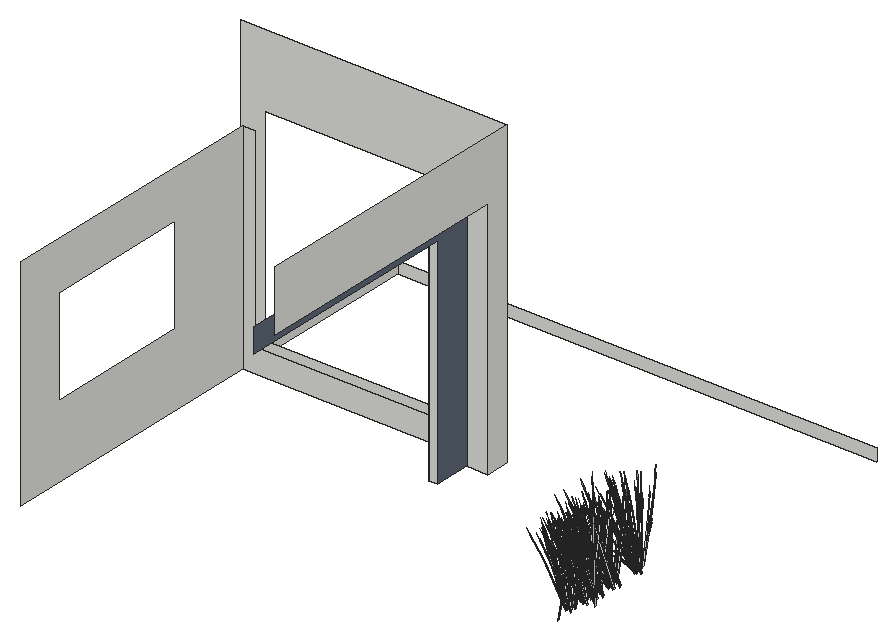
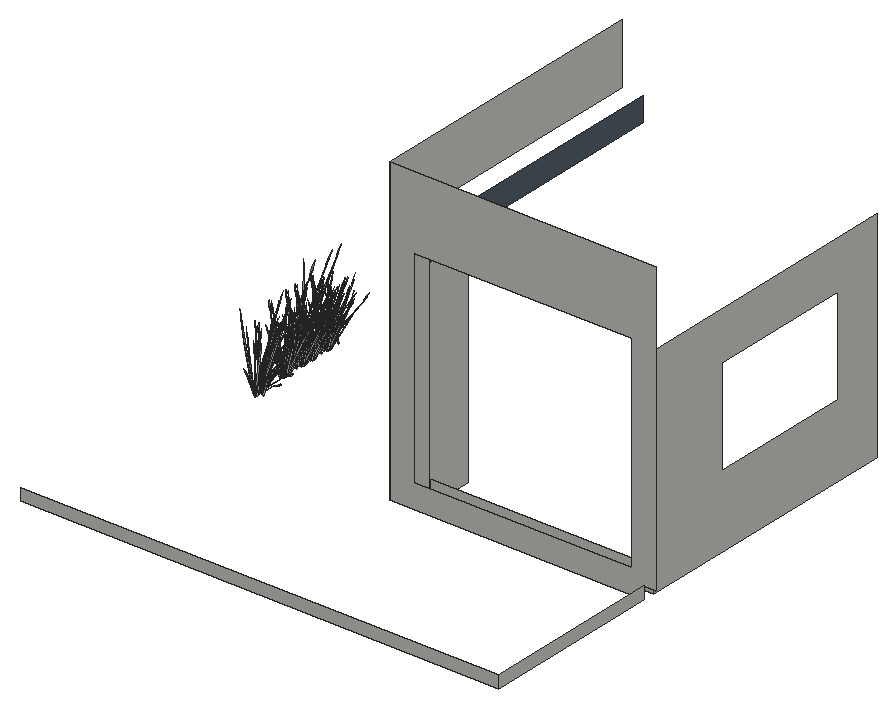
# SketchUp Ruby script. Lengths in inches.
U = 1.inch
M = Sketchup.active_model
def pt(a) = Geom::Point3d.new(a.map { |v| v * U })
def face(e, loops, mat)
  f = e.add_face(loops[0].map { |a| pt(a) })
  loops[1..].each { |l| e.add_face(l.map { |a| pt(a) }).erase! }
  f.material = f.back_material = mat if mat
  f
end
# faces: each face lists its corners as indices into pts; further lists are holes
def faces(e, pts, list, mat = nil) = list.each { |f| face(e, (f[0].is_a?(Array) ? f : [f]).map { |l| l.map { |i| pts[i] } }, mat) }
# xy, xz, yz: faces in a plane at the given z, y or x. An outline is a flat list of corners, or four numbers for a rectangle; further outlines are holes
def ring(l) = l.size == 4 ? [[l[0], l[1]], [l[2], l[1]], [l[2], l[3]], [l[0], l[3]]] : l.each_slice(2).to_a
def flat(e, list, mat, &to3) = list.each { |f| face(e, (f[0].is_a?(Array) ? f : [f]).map { |l| ring(l).map { |u, v| to3.(u, v) } }, mat) }
def xy(e, z, list, mat = nil) = flat(e, list, mat) { |x, y| [x, y, z] }
def xz(e, y, list, mat = nil) = flat(e, list, mat) { |x, z| [x, y, z] }
def yz(e, x, list, mat = nil) = flat(e, list, mat) { |y, z| [x, y, z] }
def lines(e, pts, list) = list.each { |a, b| e.add_line(pt(pts[a]), pt(pts[b])) }
# prism: a flat outline (further loops are holes) pulled along v
def prism(e, loops, v, mat = nil)
  f = face(e, loops, mat); d = Geom::Vector3d.new(v.map { |x| x * U })
  f.pushpull(f.normal.samedirection?(d) ? d.length : -d.length)
end
def box(e, o, s, mat = nil) = prism(e, [[o, [o[0] + s[0], o[1], o[2]], [o[0] + s[0], o[1] + s[1], o[2]], [o[0], o[1] + s[1], o[2]]]], [0, 0, s[2]], mat)
def at(x, y, z, deg = 0) = Geom::Transformation.translation(pt([x, y, z])) * Geom::Transformation.rotation(ORIGIN, Z_AXIS, deg.degrees)
def axes(o, x, y, z) = Geom::Transformation.new([*x, 0, *y, 0, *z, 0, *pt(o).to_a, 1])
def part(name) = M.definitions.add(name)
# library, detail: a bought-in or finely detailed component or shape, given as its bounding box
def library(name, o, s) = part(name).tap { |d| box(d.entities, o, s) }
def detail(e, o, s) = box(e.add_group.entities, o, s)
def put(e, d, t, mat = nil) = e.add_instance(d, t).tap { |i| i.material = mat if mat }
def group(e, t, mat = nil) = e.add_group.tap { |g| g.transformation = t; g.material = mat if mat }.entities
root = M.entities
M.materials.add("Denim_03_1K").color = [93, 106, 119]
M.materials.add("LightPink_Translucent").color = [144, 107, 117]
M.materials["LightPink_Translucent"].alpha = 0.75
c1 = part("blade")
p = [[2.15,0.21,22],[0,0.17,0],[0.09,0.45,0],[2.18,0.31,22],[2.29,0.31,22],[0.38,0.45,0],
  [2.48,0.24,33],[2.49,0.24,33],[2.48,0.22,33]]
faces(c1.entities,p,[[0,1,2,3],[4,5,2,3],[6,3,4,7],[8,0,3,6]])
c2 = part("seeds")
p = [[0.3,-0.1,1.38],[-0.01,-0.03,1.59],[-0.01,-0.03,0.03],[0.14,-0.07,-0.07],[0.29,-0.03,3],[0.15,0.01,3.11]]
faces(c2.entities,p,[[0,1,2,3],[1,0,4,5]],"LightPink_Translucent")
c3 = part("blade with seeds")
put(c3.entities,c1,at(0,0,0))
put(c3.entities,c2,axes([2.4,0.25,30.99],[1.5799,-0.05474,1.17369],[-0.12525,1.92788,0.29478],[-0.07173,-0.02425,1.56792]))
xz(root,405,[[162,126,166.5,234]])
xz(root,423,[[166.5,126,177,246]])
xz(root,429,[[51,126,162,126,162,138,57,138,57,234,51,234]])
xz(root,435,[[[51,126,51,132,45,132,45,276,177,276,177,126],[57,138,165,240]]])
xz(root,525,[[51,126,288,132]])
yz(root,51,[[[291,126,429,234],[315,162,387,210]],[435,126,525,132]])
yz(root,162,[[405,126,429,234]])
yz(root,166.5,[[405,126,423,126,423,246,291,246,291,234,405,234]],"Denim_03_1K")
yz(root,177,[[423,126,435,126,435,276,291,276,291,246,423,246]])
put(root,c3,axes([268.35,357.15,126.52],[0.37107,-0.01478,1.71376],[-0.24616,0.64047,0.13857],[-0.5288,-0.03961,0.73262]))
put(root,c3,axes([268.35,366.98,126.55],[0.37107,-0.01478,1.71376],[-0.24616,0.64047,0.13857],[-0.5288,-0.03961,0.73262]))
put(root,c3,axes([268.35,372.59,126.42],[0.37107,-0.01478,1.71376],[-0.24616,0.64047,0.13857],[-0.5288,-0.03961,0.73262]))
put(root,c3,axes([268.35,382.95,126.46],[0.37107,-0.01478,1.71376],[-0.24616,0.64047,0.13857],[-0.5288,-0.03961,0.73262]))
put(root,c3,axes([268.35,400.0625,125.79],[0.37107,-0.01478,1.71376],[-0.24616,0.64047,0.13857],[-0.5288,-0.03961,0.73262]))
put(root,c3,axes([268.51,358.28,126.52],[0.31041,-0.13801,1.71376],[0.26133,0.63772,0.13857],[-0.48731,0.14413,0.73262]))
put(root,c3,axes([268.51,368.1,126.55],[0.31041,-0.13801,1.71376],[0.26133,0.63772,0.13857],[-0.48731,0.14413,0.73262]))
put(root,c3,axes([268.51,373.72,126.42],[0.31041,-0.13801,1.71376],[0.26133,0.63772,0.13857],[-0.48731,0.14413,0.73262]))
put(root,c3,axes([268.51,384.08,126.46],[0.31041,-0.13801,1.71376],[0.26133,0.63772,0.13857],[-0.48731,0.14413,0.73262]))
put(root,c3,axes([268.51,401.19,125.79],[0.31041,-0.13801,1.71376],[0.26133,0.63772,0.13857],[-0.48731,0.14413,0.73262]))
put(root,c3,axes([270.29,357.62,125.99],[0.25429,-0.09438,1.77064],[0.08769,0.65901,0.13857],[-0.5508,0.08745,0.63284]))
put(root,c3,axes([270.29,367.4375,126.02],[0.25429,-0.09438,1.77064],[0.08769,0.65901,0.13857],[-0.5508,0.08745,0.63284]))
put(root,c3,axes([270.29,373.05,125.89],[0.25429,-0.09438,1.77064],[0.08769,0.65901,0.13857],[-0.5508,0.08745,0.63284]))
put(root,c3,axes([270.29,383.41,125.92],[0.25429,-0.09438,1.77064],[0.08769,0.65901,0.13857],[-0.5508,0.08745,0.63284]))
put(root,c3,axes([267.56,400.97,126.63],[-0.14609,0.08471,1.74944],[0.01243,0.61893,-0.27667],[-0.33486,0.08049,0.14031]))
put(root,c3,axes([269.46,366.38,127.66],[-0.89428,-0.01571,-0.71045],[0.06006,-0.66153,0.08574],[-0.37886,-0.06981,1.00501]))
put(root,c3,axes([269.46,382.36,127.5625],[-0.89428,-0.01571,-0.71045],[0.06006,-0.66153,0.08574],[-0.37886,-0.06981,1.00501]))
put(root,c3,axes([268.03,357.7,127.17],[-0.74348,-0.18202,-0.35414],[0.21685,-0.53102,0.4572],[-0.29933,0.04869,0.87481]))
put(root,c3,axes([268.03,367.53,127.2],[-0.74348,-0.18202,-0.35414],[0.21685,-0.53102,0.4572],[-0.29933,0.04869,0.87481]))
put(root,c3,axes([268.03,373.14,127.07],[-0.74348,-0.18202,-0.35414],[0.21685,-0.53102,0.4572],[-0.29933,0.04869,0.87481]))
put(root,c3,axes([268.03,383.5,127.11],[-0.74348,-0.18202,-0.35414],[0.21685,-0.53102,0.4572],[-0.29933,0.04869,0.87481]))
put(root,c3,axes([269.05,365.95,126.55],[0.3323,0.11241,1.71376],[-0.68769,0.4716,0.13857],[-0.42861,-0.21275,0.73262]))
put(root,c3,axes([269.05,371.5625,126.42],[0.3323,0.11241,1.71376],[-0.68769,0.4716,0.13857],[-0.42861,-0.21275,0.73262]))
put(root,c3,axes([269.05,381.92,126.46],[0.3323,0.11241,1.71376],[-0.68769,0.4716,0.13857],[-0.42861,-0.21275,0.73262]))
put(root,c3,axes([269.05,399.04,125.79],[0.3323,0.11241,1.71376],[-0.68769,0.4716,0.13857],[-0.42861,-0.21275,0.73262]))
put(root,c3,axes([265.93,401.59,126.625],[0.11417,0.0175,1.77383],[0.35319,0.57649,-0.16761],[-0.23371,0.15131,0.31391]))
put(root,c3,axes([268.54,357.97,127.33],[-0.24236,0.59349,-0.51099],[-0.83094,-0.20343,-0.3958],[-0.33455,0.05442,0.97773]))
put(root,c3,axes([268.54,367.8,127.36],[-0.24236,0.59349,-0.51099],[-0.83094,-0.20343,-0.3958],[-0.33455,0.05442,0.97773]))
put(root,c3,axes([268.54,373.41,127.23],[-0.24236,0.59349,-0.51099],[-0.83094,-0.20343,-0.3958],[-0.33455,0.05442,0.97773]))
put(root,c3,axes([268.54,383.77,127.26],[-0.24236,0.59349,-0.51099],[-0.83094,-0.20343,-0.3958],[-0.33455,0.05442,0.97773]))
put(root,c3,axes([269.17,366.51,127.36],[-0.6496,0.4322,-0.51099],[-0.5689,-0.45657,-0.3958],[-0.33005,-0.06576,0.97773]))
put(root,c3,axes([269.17,372.13,127.23],[-0.6496,0.4322,-0.51099],[-0.5689,-0.45657,-0.3958],[-0.33005,-0.06576,0.97773]))
put(root,c3,axes([269.17,382.49,127.26],[-0.6496,0.4322,-0.51099],[-0.5689,-0.45657,-0.3958],[-0.33005,-0.06576,0.97773]))
put(root,c3,axes([268.25,398.39,126.625],[0.06632,0.06511,1.77383],[-0.31973,0.58531,-0.16761],[-0.32381,0.00424,0.31391]))
put(root,c3,axes([268.99,398,126.63],[-0.19249,-0.00461,1.74944],[-0.61281,0.46055,-0.27667],[-0.32697,-0.0941,0.14031]))
put(root,c3,axes([268.2,400.55,126.65],[0.25275,-0.59491,0.48003],[0.83094,0.20343,0.3958],[-0.32677,0.03575,0.9933]))
put(root,c3,axes([268.5,357.47,127.68],[0.45012,0.59081,-0.1216],[-0.79888,0.29033,-0.67495],[-0.33665,0.07795,1.02557]))
put(root,c3,axes([268.5,372.9,127.58],[0.45012,0.59081,-0.1216],[-0.79888,0.29033,-0.67495],[-0.33665,0.07795,1.02557]))
put(root,c3,axes([268.5,383.26,127.61],[0.45012,0.59081,-0.1216],[-0.79888,0.29033,-0.67495],[-0.33665,0.07795,1.02557]))
put(root,c3,axes([268.5,400.375,126.95],[0.45012,0.59081,-0.1216],[-0.79888,0.29033,-0.67495],[-0.33665,0.07795,1.02557]))
put(root,c3,axes([269.51,356.24,127.68],[-0.0479,0.66354,-0.1216],[-0.90696,-0.01814,-0.67495],[-0.3493,-0.04609,1.02557]))
put(root,c3,axes([269.51,371.68,127.58],[-0.0479,0.66354,-0.1216],[-0.90696,-0.01814,-0.67495],[-0.3493,-0.04609,1.02557]))
put(root,c3,axes([269.51,382.04,127.61],[-0.0479,0.66354,-0.1216],[-0.90696,-0.01814,-0.67495],[-0.3493,-0.04609,1.02557]))
put(root,c3,axes([269.51,399.15,126.95],[-0.0479,0.66354,-0.1216],[-0.90696,-0.01814,-0.67495],[-0.3493,-0.04609,1.02557]))
put(root,c3,axes([268.92,366.11,127.2],[-0.50902,-0.40851,-0.35414],[0.58122,-0.38671,0.4572],[-0.29531,-0.05884,0.87481]))
put(root,c3,axes([268.92,371.72,127.07],[-0.50902,-0.40851,-0.35414],[0.58122,-0.38671,0.4572],[-0.29531,-0.05884,0.87481]))
put(root,c3,axes([268.92,382.08,127.11],[-0.50902,-0.40851,-0.35414],[0.58122,-0.38671,0.4572],[-0.29531,-0.05884,0.87481]))
put(root,c3,axes([268.14,400.39,126.64],[-0.32857,-0.44488,0.0643],[0.59916,-0.21775,0.50621],[-0.26412,0.04296,0.77189]))
put(root,c3,axes([269.64,358.71,126.52],[0.22344,-0.20048,1.71376],[0.56419,0.54113,0.13857],[-0.38697,0.24643,0.73262]))
put(root,c3,axes([269.64,368.53,126.55],[0.22344,-0.20048,1.71376],[0.56419,0.54113,0.13857],[-0.38697,0.24643,0.73262]))
put(root,c3,axes([269.64,374.15,126.42],[0.22344,-0.20048,1.71376],[0.56419,0.54113,0.13857],[-0.38697,0.24643,0.73262]))
put(root,c3,axes([269.64,384.51,126.46],[0.22344,-0.20048,1.71376],[0.56419,0.54113,0.13857],[-0.38697,0.24643,0.73262]))
put(root,c3,axes([269.64,401.62,125.79],[0.22344,-0.20048,1.71376],[0.56419,0.54113,0.13857],[-0.38697,0.24643,0.73262]))
put(root,c3,axes([268.3,359.24,127.17],[-0.77872,0.09325,-0.35414],[-0.20563,-0.53305,0.4572],[-0.22316,0.14318,0.87481]))
put(root,c3,axes([268.3,369.06,127.2],[-0.77872,0.09325,-0.35414],[-0.20563,-0.53305,0.4572],[-0.22316,0.14318,0.87481]))
put(root,c3,axes([268.3,374.67,127.07],[-0.77872,0.09325,-0.35414],[-0.20563,-0.53305,0.4572],[-0.22316,0.14318,0.87481]))
put(root,c3,axes([268.3,385.03,127.11],[-0.77872,0.09325,-0.35414],[-0.20563,-0.53305,0.4572],[-0.22316,0.14318,0.87481]))
put(root,c3,axes([268.4,402.03,126.65],[-0.22187,-0.60049,0.48003],[0.87033,-0.10422,0.3958],[-0.25651,0.14123,0.9933]))
put(root,c3,axes([268.85,399.04,127.01],[0.7388,-0.48151,0.53763],[0.63717,0.51135,0.4433],[-0.34662,-0.08882,1.11249]))
put(root,c3,axes([268.23,401.91,126.64],[-0.61415,-0.2744,0.0643],[0.35756,-0.39076,0.50621],[-0.1969,0.12633,0.77189]))
put(root,c3,axes([269.48,359.2,126.52],[0.16657,-0.22426,1.71376],[0.69879,0.4641,0.13857],[-0.31524,0.28926,0.73262]))
put(root,c3,axes([269.48,369.03,126.55],[0.16657,-0.22426,1.71376],[0.69879,0.4641,0.13857],[-0.31524,0.28926,0.73262]))
put(root,c3,axes([269.48,374.64,126.42],[0.16657,-0.22426,1.71376],[0.69879,0.4641,0.13857],[-0.31524,0.28926,0.73262]))
put(root,c3,axes([269.48,385,126.46],[0.16657,-0.22426,1.71376],[0.69879,0.4641,0.13857],[-0.31524,0.28926,0.73262]))
put(root,c3,axes([269.48,402.11,125.79],[0.16657,-0.22426,1.71376],[0.69879,0.4641,0.13857],[-0.31524,0.28926,0.73262]))
put(root,c3,axes([268.81,400.56,126.97],[0.74348,0.18202,0.35414],[-0.21685,0.53102,-0.4572],[-0.29933,0.04869,0.87481]))
put(root,c3,axes([268.94,359.3,127.33],[0.22982,0.59576,-0.51099],[-0.87033,0.10422,-0.3958],[-0.24941,0.16002,0.97773]))
put(root,c3,axes([268.94,369.12,127.36],[0.22982,0.59576,-0.51099],[-0.87033,0.10422,-0.3958],[-0.24941,0.16002,0.97773]))
put(root,c3,axes([268.94,374.73,127.23],[0.22982,0.59576,-0.51099],[-0.87033,0.10422,-0.3958],[-0.24941,0.16002,0.97773]))
put(root,c3,axes([268.94,385.1,127.26],[0.22982,0.59576,-0.51099],[-0.87033,0.10422,-0.3958],[-0.24941,0.16002,0.97773]))
put(root,c3,axes([269.19,399.04,126.64],[0.04505,-0.49615,0.0643],[0.68022,0.0136,0.50621],[-0.26056,-0.05192,0.77189]))
put(root,c3,axes([267.58,403.28,126.63],[-0.02224,0.12912,1.74944],[0.63107,0.44917,-0.27667],[-0.16521,0.21241,0.14031]))
put(root,c3,axes([271.28,398.18,127.34],[-0.59706,0.6255,-0.13619],[-0.86465,-0.36036,-0.75594],[-0.30056,-0.17672,1.14864]))
put(root,c3,axes([269.65,399.41,126.97],[0.50902,0.40851,0.35414],[-0.58122,0.38671,-0.4572],[-0.29531,-0.05884,0.87481]))
put(root,c3,axes([271.02,365.6,127.66],[-0.76283,-0.31537,-0.71045],[0.54213,-0.55263,0.08574],[-0.27638,-0.1883,1.00501]))
put(root,c3,axes([271.02,381.58,127.5625],[-0.76283,-0.31537,-0.71045],[0.54213,-0.55263,0.08574],[-0.27638,-0.1883,1.00501]))
put(root,c3,axes([270.66,365.62,127.36],[-0.88277,0.1551,-0.51099],[-0.15442,-0.58737,-0.3958],[-0.23711,-0.16832,0.97773]))
put(root,c3,axes([270.66,371.23,127.23],[-0.88277,0.1551,-0.51099],[-0.15442,-0.58737,-0.3958],[-0.23711,-0.16832,0.97773]))
put(root,c3,axes([270.66,381.59,127.26],[-0.88277,0.1551,-0.51099],[-0.15442,-0.58737,-0.3958],[-0.23711,-0.16832,0.97773]))
put(root,c3,axes([268.53,358.87,127.68],[0.82753,0.35977,-0.1216],[-0.47675,0.52101,-0.67495],[-0.2338,0.18111,1.02557]))
put(root,c3,axes([268.53,374.31,127.58],[0.82753,0.35977,-0.1216],[-0.47675,0.52101,-0.67495],[-0.2338,0.18111,1.02557]))
put(root,c3,axes([268.53,384.67,127.61],[0.82753,0.35977,-0.1216],[-0.47675,0.52101,-0.67495],[-0.2338,0.18111,1.02557]))
put(root,c3,axes([268.53,401.78,126.95],[0.82753,0.35977,-0.1216],[-0.47675,0.52101,-0.67495],[-0.2338,0.18111,1.02557]))
put(root,c3,axes([268.93,401.83,126.97],[0.77872,-0.09325,0.35414],[0.20563,0.53305,-0.4572],[-0.22316,0.14318,0.87481]))
put(root,c3,axes([271.05,396.69,126.625],[-0.01669,0.07821,1.77383],[-0.82314,0.28383,-0.16761],[-0.24223,-0.14508,0.31391]))
put(root,c3,axes([270.42,365.29,126.55],[0.2045,0.20949,1.71376],[-0.94495,0.17636,0.13857],[-0.21357,-0.32887,0.73262]))
put(root,c3,axes([270.42,370.91,126.42],[0.2045,0.20949,1.71376],[-0.94495,0.17636,0.13857],[-0.21357,-0.32887,0.73262]))
put(root,c3,axes([270.42,381.27,126.46],[0.2045,0.20949,1.71376],[-0.94495,0.17636,0.13857],[-0.21357,-0.32887,0.73262]))
put(root,c3,axes([270.42,398.38,125.79],[0.2045,0.20949,1.71376],[-0.94495,0.17636,0.13857],[-0.21357,-0.32887,0.73262]))
put(root,c3,axes([269.67,403.25,126.65],[-0.63704,-0.44518,0.48003],[0.67652,-0.38394,0.3958],[-0.11751,0.20886,0.9933]))
put(root,c3,axes([270.75,365.18,127.2],[-0.13817,-0.52554,-0.35414],[0.78985,-0.13877,0.4572],[-0.21215,-0.1506,0.87481]))
put(root,c3,axes([270.75,370.8,127.07],[-0.13817,-0.52554,-0.35414],[0.78985,-0.13877,0.4572],[-0.21215,-0.1506,0.87481]))
put(root,c3,axes([270.75,381.16,127.11],[-0.13817,-0.52554,-0.35414],[0.78985,-0.13877,0.4572],[-0.21215,-0.1506,0.87481]))
put(root,c3,axes([269.4375,403.2,126.64],[-0.73517,-0.0304,0.0643],[0.02016,-0.45906,0.50621],[-0.07693,0.17585,0.77189]))
put(root,c3,axes([269.67,360.47,127.17],[-0.60531,0.34352,-0.35414],[-0.573,-0.39225,0.4572],[-0.08718,0.19929,0.87481]))
put(root,c3,axes([269.67,370.29,127.2],[-0.60531,0.34352,-0.35414],[-0.573,-0.39225,0.4572],[-0.08718,0.19929,0.87481]))
put(root,c3,axes([269.67,375.9,127.07],[-0.60531,0.34352,-0.35414],[-0.573,-0.39225,0.4572],[-0.08718,0.19929,0.87481]))
put(root,c3,axes([269.67,386.27,127.11],[-0.60531,0.34352,-0.35414],[-0.573,-0.39225,0.4572],[-0.08718,0.19929,0.87481]))
put(root,c3,axes([271.22,398.7,126.97],[0.13817,0.52554,0.35414],[-0.78985,0.13877,-0.4572],[-0.21215,-0.1506,0.87481]))
put(root,c3,axes([267.51,404.6,126.625],[0.10149,-0.03939,1.77383],[0.83886,0.26202,-0.16761],[-0.01971,0.21816,0.31391]))
put(root,c3,axes([272.84,369.17,126],[0.77308,0.2631,1.51261],[-0.75736,0.56681,0.59816],[-0.33924,-0.33594,1.26806]))
put(root,c3,axes([272.84,374.78,125.875],[0.77308,0.2631,1.51261],[-0.75736,0.56681,0.59816],[-0.33924,-0.33594,1.26806]))
put(root,c3,axes([272.84,385.14,125.91],[0.77308,0.2631,1.51261],[-0.75736,0.56681,0.59816],[-0.33924,-0.33594,1.26806]))
put(root,c3,axes([270.07,360.11,127.98],[-0.02328,0.60353,-0.7886],[-0.98022,-0.04053,0.09517],[-0.10344,0.25568,1.11556]))
put(root,c3,axes([270.07,369.93,128.01],[-0.02328,0.60353,-0.7886],[-0.98022,-0.04053,0.09517],[-0.10344,0.25568,1.11556]))
put(root,c3,axes([270.07,375.54,127.89],[-0.02328,0.60353,-0.7886],[-0.98022,-0.04053,0.09517],[-0.10344,0.25568,1.11556]))
put(root,c3,axes([270.07,385.9,127.92],[-0.02328,0.60353,-0.7886],[-0.98022,-0.04053,0.09517],[-0.10344,0.25568,1.11556]))
put(root,c3,axes([270.87,398.08,127.01],[0.99656,-0.1677,0.53763],[0.17295,0.65785,0.4433],[-0.23438,-0.19388,1.11249]))
put(root,c3,axes([271.09,398.22,126.64],[0.4066,-0.41448,0.0643],[0.57901,0.24131,0.50621],[-0.18719,-0.13288,0.77189]))
put(root,c3,axes([269.74,350.42,125.6875],[0.01966,-0.33682,1.54345],[0.88405,0.17791,0.21329],[-0.0766,0.35897,0.72882]))
put(root,c3,axes([269.74,360.96,126.01],[0.01966,-0.33682,1.54345],[0.88405,0.17791,0.21329],[-0.0766,0.35897,0.72882]))
put(root,c3,axes([269.74,370.78,126.04],[0.01966,-0.33682,1.54345],[0.88405,0.17791,0.21329],[-0.0766,0.35897,0.72882]))
put(root,c3,axes([269.74,376.39,125.91],[0.01966,-0.33682,1.54345],[0.88405,0.17791,0.21329],[-0.0766,0.35897,0.72882]))
put(root,c3,axes([269.74,386.75,125.94],[0.01966,-0.33682,1.54345],[0.88405,0.17791,0.21329],[-0.0766,0.35897,0.72882]))
put(root,c3,axes([271.98,396.99,126.63],[-0.13683,-0.09148,1.74944],[-0.91315,0.058,-0.27667],[-0.14574,-0.2188,0.14031]))
put(root,c3,axes([270.27,360.31,127.65],[0.64041,0.4384,-0.5672],[-0.67652,0.38394,-0.43934],[-0.09744,0.22274,1.08528]))
put(root,c3,axes([270.27,370.13,127.68],[0.64041,0.4384,-0.5672],[-0.67652,0.38394,-0.43934],[-0.09744,0.22274,1.08528]))
put(root,c3,axes([270.27,375.74,127.55],[0.64041,0.4384,-0.5672],[-0.67652,0.38394,-0.43934],[-0.09744,0.22274,1.08528]))
put(root,c3,axes([270.27,386.1,127.59],[0.64041,0.4384,-0.5672],[-0.67652,0.38394,-0.43934],[-0.09744,0.22274,1.08528]))
put(root,c3,axes([269.98,402.89,126.97],[0.60531,-0.34352,0.35414],[0.573,0.39225,-0.4572],[-0.08718,0.19929,0.87481]))
put(root,c3,axes([274.04,367.91,125.52],[-0.02444,-0.61432,1.41272],[1.10603,0.15924,0.59816],[-0.26159,0.33615,1.3335]))
put(root,c3,axes([269.6,402.99,127.3125],[0.98321,0.03233,-0.13498],[-0.02687,0.61208,-0.74919],[-0.0683,0.23574,1.13838]))
put(root,c3,axes([273.37,370.93,127.58],[-0.87543,0.30377,-0.1216],[-0.4302,-0.53915,-0.67495],[-0.1155,-0.2272,1.02557]))
put(root,c3,axes([273.37,381.29,127.61],[-0.87543,0.30377,-0.1216],[-0.4302,-0.53915,-0.67495],[-0.1155,-0.2272,1.02557]))
put(root,c3,axes([273.37,398.4,126.95],[-0.87543,0.30377,-0.1216],[-0.4302,-0.53915,-0.67495],[-0.1155,-0.2272,1.02557]))
put(root,c3,axes([272.62,365.34,127.36],[-0.87941,-0.16356,-0.51099],[0.30143,-0.56078,-0.3958],[-0.08064,-0.22578,0.97773]))
put(root,c3,axes([272.62,370.96,127.23],[-0.87941,-0.16356,-0.51099],[0.30143,-0.56078,-0.3958],[-0.08064,-0.22578,0.97773]))
put(root,c3,axes([272.62,381.32,127.26],[-0.87941,-0.16356,-0.51099],[0.30143,-0.56078,-0.3958],[-0.08064,-0.22578,0.97773]))
